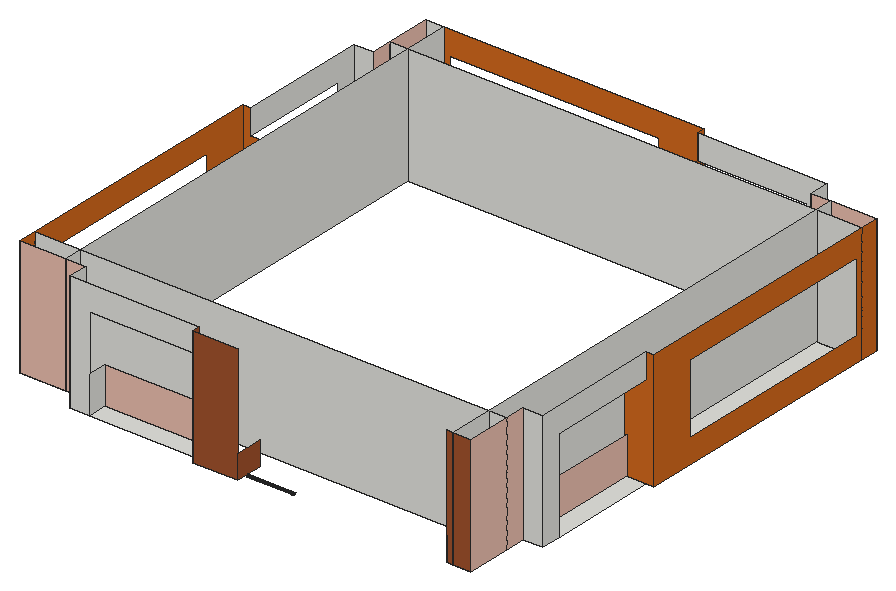
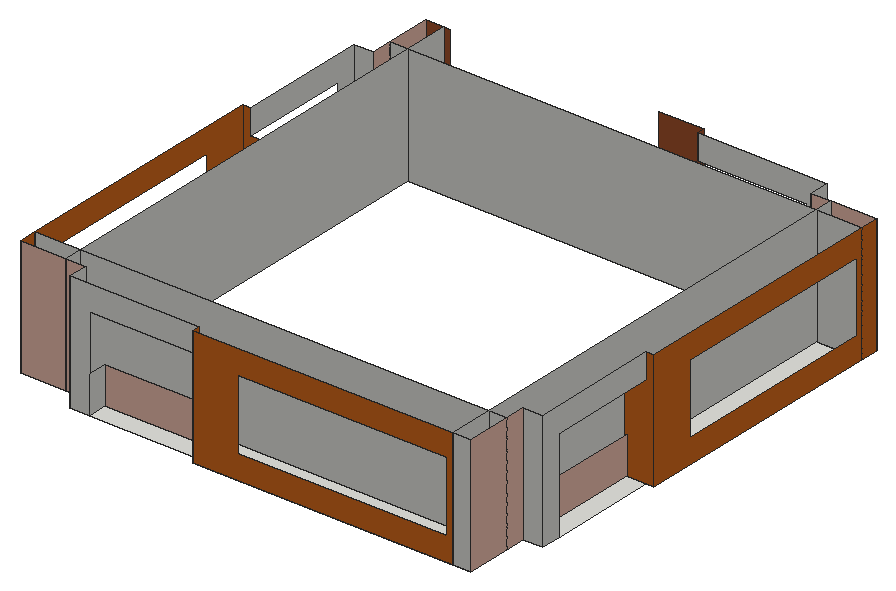
# SketchUp Ruby script. Lengths in inches.
U = 1.inch
M = Sketchup.active_model
def pt(a) = Geom::Point3d.new(a.map { |v| v * U })
def face(e, loops, mat)
  f = e.add_face(loops[0].map { |a| pt(a) })
  loops[1..].each { |l| e.add_face(l.map { |a| pt(a) }).erase! }
  f.material = f.back_material = mat if mat
  f
end
# faces: each face lists its corners as indices into pts; further lists are holes
def faces(e, pts, list, mat = nil) = list.each { |f| face(e, (f[0].is_a?(Array) ? f : [f]).map { |l| l.map { |i| pts[i] } }, mat) }
# xy, xz, yz: faces in a plane at the given z, y or x. An outline is a flat list of corners, or four numbers for a rectangle; further outlines are holes
def ring(l) = l.size == 4 ? [[l[0], l[1]], [l[2], l[1]], [l[2], l[3]], [l[0], l[3]]] : l.each_slice(2).to_a
def flat(e, list, mat, &to3) = list.each { |f| face(e, (f[0].is_a?(Array) ? f : [f]).map { |l| ring(l).map { |u, v| to3.(u, v) } }, mat) }
def xy(e, z, list, mat = nil) = flat(e, list, mat) { |x, y| [x, y, z] }
def xz(e, y, list, mat = nil) = flat(e, list, mat) { |x, z| [x, y, z] }
def yz(e, x, list, mat = nil) = flat(e, list, mat) { |y, z| [x, y, z] }
def lines(e, pts, list) = list.each { |a, b| e.add_line(pt(pts[a]), pt(pts[b])) }
# prism: a flat outline (further loops are holes) pulled along v
def prism(e, loops, v, mat = nil)
  f = face(e, loops, mat); d = Geom::Vector3d.new(v.map { |x| x * U })
  f.pushpull(f.normal.samedirection?(d) ? d.length : -d.length)
end
def box(e, o, s, mat = nil) = prism(e, [[o, [o[0] + s[0], o[1], o[2]], [o[0] + s[0], o[1] + s[1], o[2]], [o[0], o[1] + s[1], o[2]]]], [0, 0, s[2]], mat)
def at(x, y, z, deg = 0) = Geom::Transformation.translation(pt([x, y, z])) * Geom::Transformation.rotation(ORIGIN, Z_AXIS, deg.degrees)
def axes(o, x, y, z) = Geom::Transformation.new([*x, 0, *y, 0, *z, 0, *pt(o).to_a, 1])
def part(name) = M.definitions.add(name)
# library, detail: a bought-in or finely detailed component or shape, given as its bounding box
def library(name, o, s) = part(name).tap { |d| box(d.entities, o, s) }
def detail(e, o, s) = box(e.add_group.entities, o, s)
def put(e, d, t, mat = nil) = e.add_instance(d, t).tap { |i| i.material = mat if mat }
def group(e, t, mat = nil) = e.add_group.tap { |g| g.transformation = t; g.material = mat if mat }.entities
root = M.entities
M.materials.add("[0041_Chocolate]").color = [210, 105, 30]
M.materials.add("[0042_Sienna]").color = [160, 82, 45]
M.materials.add("[0119_RosyBrown]").color = [234, 190, 174]
xy(root,1140,[[1434.3125,12.8125,1488,150.5],[306.65,36.8125,641.22,96.8125],[48,96.8125,185.6875,150.5],[48,150.5,185.6875,150.5,185.6875,1399.125,132,1399.125,132,1338.16,72,1338.16,72,1278.16,132,1278.16,132,943.59,48,943.59],[1434.3125,150.5,1488,150.5,1488,211.46,1548,211.46,1548,271.47,1488,271.47,1488,606.03,1572,606.03,1572,1399.125,1434.3125,1399.125],
  [1488,271.47,1548,606.03],[72,943.59,132,1278.16],[132,1399.125,185.6875,1536.8125],[185.6875,1399.125,1434.3125,1399.125,1434.3125,1452.8125,1373.35,1452.8125,1373.35,1512.8125,1313.35,1512.8125,1313.35,1452.8125,978.78,1452.8125,978.78,1536.8125,185.6875,1536.8125],[1434.3125,1399.125,1572,1452.8125],
  [978.78,1452.8125,1313.35,1512.8125]])
xz(root,12.8125,[[641.22,1140,778.64,1500],[1414.89,1140,1434.3125,1500],[1434.3125,1140,1488,1500]],"[0042_Sienna]")
xz(root,36.8125,[[246.65,1140,306.65,1140,306.65,1422.625,641.22,1422.625,641.22,1500,246.65,1500]])
xz(root,96.8125,[[48,1140,185.6875,1500],[185.6875,1140,246.65,1500],[306.65,1140,641.22,1253.76]],"[0119_RosyBrown]")
xz(root,150.5,[[48,1140,1488,1500]])
xz(root,211.46,[[1488,1140,1548,1500]])
xz(root,271.47,[[1488,1140,1548,1253.76]])
xz(root,606.03,[[1488,1140,1572,1140,1572,1500,1548,1500,1548,1422.625,1482,1422.625,1482,1253.76,1488,1253.76]],"[0041_Chocolate]")
xz(root,943.59,[[48,1140,48,1500,72,1500,72,1422.625,138,1422.625,138,1253.76,132,1253.76,132,1140]],"[0041_Chocolate]")
xz(root,1278.16,[[72,1140,132,1253.76]])
xz(root,1338.16,[[72,1140,132,1500]])
xz(root,1399.125,[[132,1140,1572,1500]])
xz(root,1452.8125,[[978.78,1140,1313.35,1253.76],[1373.35,1140,1434.3125,1500],[1434.3125,1140,1572,1500]],"[0119_RosyBrown]")
xz(root,1512.8125,[[1313.35,1140,1313.35,1422.625,978.78,1422.625,978.78,1500,1373.35,1500,1373.35,1140]])
xz(root,1536.8125,[[132,1140,185.6875,1500]])
xz(root,1536.8125,[[[185.6875,1140,978.78,1500],[205.11,1213.11,841.36,1426.89]]],"[0041_Chocolate]")
yz(root,48,[[96.8125,1140,150.5,1500],[[150.5,1140,943.59,1500],[169.92,1213.11,806.17,1426.89]]],"[0041_Chocolate]")
yz(root,72,[[1278.16,1140,1278.16,1422.625,943.59,1422.625,943.59,1500,1338.16,1500,1338.16,1140]])
yz(root,132,[[943.59,1140,1278.16,1253.76],[1338.16,1140,1399.125,1500],[1399.125,1140,1536.8125,1500]],"[0119_RosyBrown]")
yz(root,185.6875,[[96.8125,1140,1536.8125,1500]])
yz(root,246.65,[[36.8125,1140,96.8125,1500]])
yz(root,306.65,[[36.8125,1140,96.8125,1253.76]])
yz(root,641.22,[[12.8125,1140,12.8125,1500,36.8125,1500,36.8125,1422.625,102.8125,1422.625,102.8125,1253.76,96.8125,1253.76,96.8125,1140]],"[0042_Sienna]")
yz(root,778.64,[[48.34,1134.02,49.29,1134.14,50.18,1134.51,50.95,1135.1,51.53,1135.86,51.9,1136.75,52.03,1137.7,51.9,1138.66,51.53,1139.55,51.19,1140,45.49,1140,45.15,1139.55,44.78,1138.66,44.65,1137.7,44.78,1136.75,45.15,1135.86,45.73,1135.1,46.5,1134.51,47.38,1134.14],[12.8125,1140,45.49,1140,45.73,1140.3125,46.5,1140.9,47.38,1141.27,48.34,1141.39,49.29,1141.27,50.18,1140.9,50.95,1140.3125,51.19,1140,96.8125,1140,96.8125,1213.11,49.67,1213.11,50.18,1212.9,50.95,1212.3125,51.53,1211.55,51.9,1210.66,52.03,1209.7,51.9,1208.75,51.53,1207.86,50.95,1207.1,50.18,1206.51,49.29,1206.14,48.34,1206.02,47.38,1206.14,46.5,1206.51,45.73,1207.1,45.15,1207.86,44.78,1208.75,44.65,1209.7,44.78,1210.66,45.15,1211.55,45.73,1212.3125,46.5,1212.9,47.01,1213.11,12.8125,1213.11],[45.49,1140,51.19,1140,50.95,1140.3125,50.18,1140.9,49.29,1141.27,48.34,1141.39,47.38,1141.27,46.5,1140.9,45.73,1140.3125]],"[0042_Sienna]")
yz(root,978.78,[[1452.8125,1140,1536.8125,1140,1536.8125,1500,1512.8125,1500,1512.8125,1422.625,1446.8125,1422.625,1446.8125,1253.76,1452.8125,1253.76]],"[0041_Chocolate]")
yz(root,1313.35,[[1452.8125,1140,1512.8125,1253.76]])
yz(root,1373.35,[[1452.8125,1140,1512.8125,1500]])
yz(root,1414.89,[[12.8125,1140,96.8125,1213.11]],"[0042_Sienna]")
yz(root,1434.3125,[[12.8125,1140,1452.8125,1500]])
yz(root,1488,[[12.8125,1140,150.5,1500],[150.5,1140,211.46,1500],[271.47,1140,606.03,1253.76]],"[0119_RosyBrown]")
yz(root,1548,[[211.46,1140,271.47,1140,271.47,1422.625,606.03,1422.625,606.03,1500,211.46,1500]])
yz(root,1572,[[[606.03,1140,1399.125,1500],[743.45,1213.11,1379.7,1426.89]],[1399.125,1140,1452.8125,1500]],"[0041_Chocolate]")
p = [[922.01,48.34,1134.02],[922.01,47.38,1134.14],[778.64,47.38,1134.14],[778.64,48.34,1134.02],[922.01,49.29,1134.14],[778.64,49.29,1134.14],
  [922.01,46.5,1134.51],[778.64,46.5,1134.51],[922.01,50.18,1134.51],[778.64,50.18,1134.51],[922.01,45.73,1135.1],[778.64,45.73,1135.1],
  [922.01,50.95,1135.1],[778.64,50.95,1135.1],[922.01,45.15,1135.86],[778.64,45.15,1135.86],[922.01,51.53,1135.86],[778.64,51.53,1135.86],
  [922.01,44.78,1136.75],[778.64,44.78,1136.75],[922.01,51.9,1136.75],[778.64,51.9,1136.75],[922.01,44.65,1137.7],[778.64,44.65,1137.7],
  [922.01,52.03,1137.7],[778.64,52.03,1137.7],[922.01,44.78,1138.66],[778.64,44.78,1138.66],[922.01,51.9,1138.66],[778.64,51.9,1138.66],
  [922.01,45.15,1139.55],[778.64,45.15,1139.55],[922.01,51.53,1139.55],[778.64,51.53,1139.55],[922.01,45.73,1140.3125],[778.64,45.73,1140.3125],
  [778.64,45.49,1140],[922.01,50.95,1140.3125],[778.64,51.19,1140],[778.64,50.95,1140.3125],[922.01,46.5,1140.9],[778.64,46.5,1140.9],
  [922.01,50.18,1140.9],[778.64,50.18,1140.9]]
faces(root,p,[[0,1,2,3],[4,0,3,5],[1,6,7,2],[8,4,5,9],[6,10,11,7],[12,8,9,13],[10,14,15,11],[16,12,13,17],
  [14,18,19,15],[20,16,17,21],[18,22,23,19],[24,20,21,25],[22,26,27,23],[28,24,25,29],[26,30,31,27],[32,28,29,33],
  [30,34,35,36,31],[37,32,33,38,39],[34,40,41,35],[42,37,39,43]])
